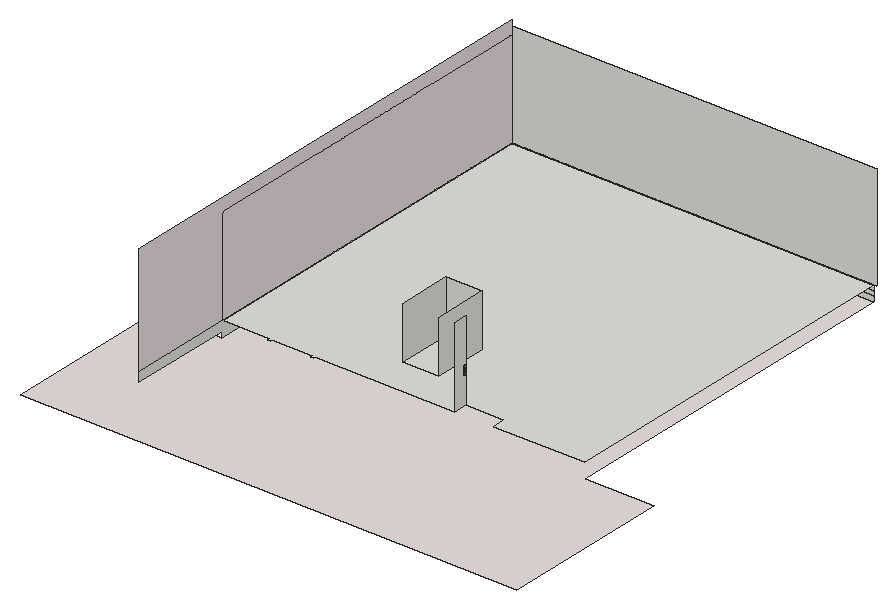
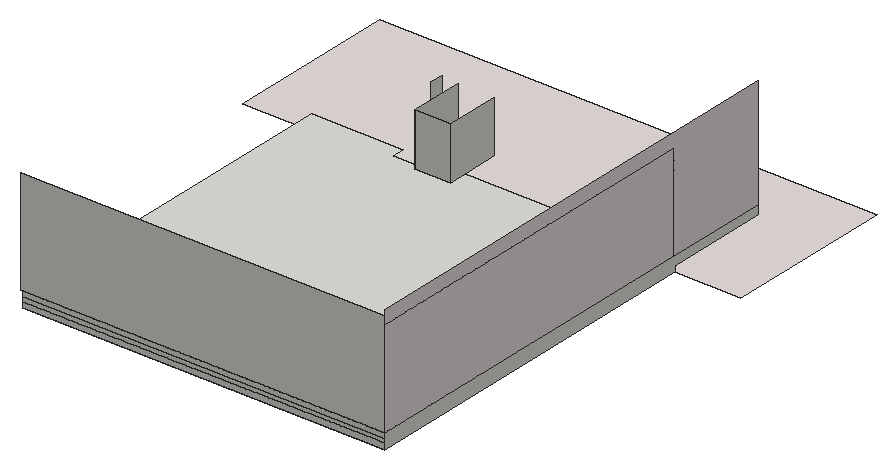
# SketchUp Ruby script. Lengths in inches.
U = 1.inch
M = Sketchup.active_model
def pt(a) = Geom::Point3d.new(a.map { |v| v * U })
def face(e, loops, mat)
  f = e.add_face(loops[0].map { |a| pt(a) })
  loops[1..].each { |l| e.add_face(l.map { |a| pt(a) }).erase! }
  f.material = f.back_material = mat if mat
  f
end
# faces: each face lists its corners as indices into pts; further lists are holes
def faces(e, pts, list, mat = nil) = list.each { |f| face(e, (f[0].is_a?(Array) ? f : [f]).map { |l| l.map { |i| pts[i] } }, mat) }
# xy, xz, yz: faces in a plane at the given z, y or x. An outline is a flat list of corners, or four numbers for a rectangle; further outlines are holes
def ring(l) = l.size == 4 ? [[l[0], l[1]], [l[2], l[1]], [l[2], l[3]], [l[0], l[3]]] : l.each_slice(2).to_a
def flat(e, list, mat, &to3) = list.each { |f| face(e, (f[0].is_a?(Array) ? f : [f]).map { |l| ring(l).map { |u, v| to3.(u, v) } }, mat) }
def xy(e, z, list, mat = nil) = flat(e, list, mat) { |x, y| [x, y, z] }
def xz(e, y, list, mat = nil) = flat(e, list, mat) { |x, z| [x, y, z] }
def yz(e, x, list, mat = nil) = flat(e, list, mat) { |y, z| [x, y, z] }
def lines(e, pts, list) = list.each { |a, b| e.add_line(pt(pts[a]), pt(pts[b])) }
# prism: a flat outline (further loops are holes) pulled along v
def prism(e, loops, v, mat = nil)
  f = face(e, loops, mat); d = Geom::Vector3d.new(v.map { |x| x * U })
  f.pushpull(f.normal.samedirection?(d) ? d.length : -d.length)
end
def box(e, o, s, mat = nil) = prism(e, [[o, [o[0] + s[0], o[1], o[2]], [o[0] + s[0], o[1] + s[1], o[2]], [o[0], o[1] + s[1], o[2]]]], [0, 0, s[2]], mat)
def at(x, y, z, deg = 0) = Geom::Transformation.translation(pt([x, y, z])) * Geom::Transformation.rotation(ORIGIN, Z_AXIS, deg.degrees)
def axes(o, x, y, z) = Geom::Transformation.new([*x, 0, *y, 0, *z, 0, *pt(o).to_a, 1])
def part(name) = M.definitions.add(name)
# library, detail: a bought-in or finely detailed component or shape, given as its bounding box
def library(name, o, s) = part(name).tap { |d| box(d.entities, o, s) }
def detail(e, o, s) = box(e.add_group.entities, o, s)
def put(e, d, t, mat = nil) = e.add_instance(d, t).tap { |i| i.material = mat if mat }
def group(e, t, mat = nil) = e.add_group.tap { |g| g.transformation = t; g.material = mat if mat }.entities
root = M.entities
M.materials.add("Generic\#9").color = [233, 223, 223]
M.materials.add("Material \#1").color = [140, 140, 140]
c1 = library("3DGeom~4_Defintion",[-18.02,-499.97,-221.16],[36.04,1000,262.12])
c2 = part("3DGeom~5_Defintion")
xy(c2.entities,-225.24,[[-0.79,-499.98,-2.33,-499.64,7.45,-496.14],[-0.79,-499.98,7.45,-496.14,1.58,-499.88],[1.58,-499.88,7.45,-496.14,3.84,-499.16],[-2.33,-499.64,7.4,-485.75,7.45,-496.14],[3.84,-499.16,7.45,-496.14,5.85,-497.89],
  [7.45,-496.14,7.4,-485.75,8.24,-487.08],[7.45,-496.14,8.24,-487.08,8.96,-489.34],[7.45,-496.14,8.96,-489.34,9.0625,-491.71],[7.45,-496.14,9.0625,-491.71,8.55,-494.03],[-7.4,-496.08,-8.24,-494.76,2.32,-482.2],
  [-8.24,-494.76,-8.96,-492.5,2.32,-482.2],[-8.96,-492.5,-9.0625,-490.125,2.32,-482.2],[-9.0625,-490.125,-8.55,-487.81,2.32,-482.2],[-8.55,-487.81,-7.45,-485.7,2.32,-482.2],[-7.45,-485.7,-5.85,-483.95,2.32,-482.2],
  [-5.85,-483.95,-3.84,-482.68,2.32,-482.2],[-3.84,-482.68,-1.58,-481.96,2.32,-482.2],[2.32,-482.2,-1.58,-481.96,0.79,-481.86],[0,481.82,-2.35,482.13,-6.92,496.71],[0,481.82,-6.92,496.71,1.55,482.04],
  [-2.35,482.13,-4.55,483.04,-6.92,496.71],[-4.55,483.04,-6.43,484.49,-6.92,496.71],[-6.43,484.49,-7.88,486.37,-6.92,496.71],[6.92,485.12,-1.55,499.8125,7.88,495.47],[6.92,485.12,7.88,495.47,7.88,486.37],
  [-7.88,486.37,-8.79,488.57,-6.92,496.71],[7.88,486.37,7.88,495.47,8.79,488.57],[-8.79,488.57,-9.1,490.92,-6.92,496.71],[8.79,488.57,7.88,495.47,9.1,490.92],[-9.1,490.92,-8.79,493.28,-6.92,496.71],
  [9.1,490.92,7.88,495.47,8.79,493.28],[-8.79,493.28,-7.88,495.47,-6.92,496.71],[7.88,495.47,-1.55,499.8125,0,500.02],[7.88,495.47,0,500.02,2.35,499.71],[7.88,495.47,2.35,499.71,4.55,498.8],
  [7.88,495.47,4.55,498.8,6.43,497.35]],"Material \#1")
xy(c2.entities,-221.57,[[-2.33,-499.64,-5.22,-498.37,7.4,-485.75],[-5.22,-498.37,-7.4,-496.08,5.22,-483.47],[-5.22,-498.37,5.22,-483.47,7.4,-485.75],[-7.4,-496.08,2.32,-482.2,5.22,-483.47],[1.55,482.04,-6.92,496.71,-4.55,498.8],
  [1.55,482.04,-4.55,498.8,4.55,483.04],[4.55,483.04,-4.55,498.8,-1.55,499.8125],[4.55,483.04,-1.55,499.8125,6.92,485.12]],"Material \#1")
xy(c2.entities,38.05,[[-2.33,-499.64,7.4,-485.75,-5.22,-498.37],[-5.22,-498.37,5.22,-483.47,-7.4,-496.08],[-5.22,-498.37,7.4,-485.75,5.22,-483.47],[-7.4,-496.08,5.22,-483.47,2.32,-482.2],[1.55,482.04,-4.55,498.8,-6.92,496.71],
  [1.55,482.04,4.55,483.04,-4.55,498.8],[4.55,483.04,-1.55,499.8125,-4.55,498.8],[4.55,483.04,6.92,485.12,-1.55,499.8125]],"Material \#1")
xy(c2.entities,41.72,[[-0.79,-499.98,7.45,-496.14,-2.33,-499.64],[-0.79,-499.98,1.58,-499.88,7.45,-496.14],[1.58,-499.88,3.84,-499.16,7.45,-496.14],[-2.33,-499.64,7.45,-496.14,7.4,-485.75],[3.84,-499.16,5.85,-497.89,7.45,-496.14],
  [7.45,-496.14,8.24,-487.08,7.4,-485.75],[7.45,-496.14,8.55,-494.03,9.0625,-491.71],[7.45,-496.14,8.96,-489.34,8.24,-487.08],[7.45,-496.14,9.0625,-491.71,8.96,-489.34],[-7.4,-496.08,2.32,-482.2,-8.24,-494.76],
  [-8.24,-494.76,2.32,-482.2,-8.96,-492.5],[-8.96,-492.5,2.32,-482.2,-9.0625,-490.125],[-9.0625,-490.125,2.32,-482.2,-8.55,-487.81],[-8.55,-487.81,2.32,-482.2,-7.45,-485.7],[-7.45,-485.7,2.32,-482.2,-5.85,-483.95],
  [-5.85,-483.95,2.32,-482.2,-3.84,-482.68],[-3.84,-482.68,2.32,-482.2,-1.58,-481.96],[2.32,-482.2,0.79,-481.86,-1.58,-481.96],[0,481.82,-6.92,496.71,-2.35,482.13],[0,481.82,1.55,482.04,-6.92,496.71],
  [-2.35,482.13,-6.92,496.71,-4.55,483.04],[-4.55,483.04,-6.92,496.71,-6.43,484.49],[-6.43,484.49,-6.92,496.71,-7.88,486.37],[6.92,485.12,7.88,495.47,-1.55,499.8125],[6.92,485.12,7.88,486.37,7.88,495.47],
  [-7.88,486.37,-6.92,496.71,-8.79,488.57],[7.88,486.37,8.79,488.57,7.88,495.47],[-8.79,488.57,-6.92,496.71,-9.1,490.92],[8.79,488.57,9.1,490.92,7.88,495.47],[-9.1,490.92,-6.92,496.71,-8.79,493.28],
  [9.1,490.92,8.79,493.28,7.88,495.47],[-8.79,493.28,-6.92,496.71,-7.88,495.47],[7.88,495.47,0,500.02,-1.55,499.8125],[7.88,495.47,2.35,499.71,0,500.02],[7.88,495.47,4.55,498.8,2.35,499.71],
  [7.88,495.47,6.43,497.35,4.55,498.8]],"Material \#1")
c3 = library("3DGeom~12_Defintion",[-95.68,-755.75,-830.03],[191.36,191.37,1000])
c4 = part("3DGeom~10_Defintion")
yz(c4.entities,-68.96,[[-797.08,-844.83,-797.08,-827.59,-922.41,-827.59],[-922.41,-844.83,-797.08,-844.83,-922.41,-827.59]],"Material \#1")
yz(c4.entities,68.97,[[-922.41,-844.83,-797.08,-827.59,-797.08,-844.83],[-922.41,-844.83,-922.41,-827.59,-797.08,-827.59],[-797.08,137.93,-922.41,155.17,-797.08,155.17],[-922.41,137.93,-922.41,155.17,-797.08,137.93]],"Material \#1")
p = [[-15.8,-989.55,-844.83],[-15.8,-989.55,-827.59],[0,-991.38,-827.59],[0,-991.38,-844.83],[15.8,-989.55,-827.59],[15.8,-989.55,-844.83],
  [-30.32,-984.36,-844.83],[-30.32,-984.36,-827.59],[30.31,-984.36,-827.59],[30.31,-984.36,-844.83],[-43.12,-976.21,-844.83],[-43.12,-976.21,-827.59],
  [43.12,-976.21,-827.59],[43.12,-976.21,-844.83],[-53.81,-965.53,-844.83],[-53.81,-965.53,-827.59],[53.8,-965.53,-827.59],[53.8,-965.53,-844.83],
  [-61.95,-952.73,-844.83],[-61.95,-952.73,-827.59],[53.8,-965.53,-827.59],[61.95,-952.73,-827.59],[61.95,-952.73,-844.83],[-67.15,-938.21,-844.83],
  [-67.15,-938.21,-827.59],[67.14,-938.21,-827.59],[67.14,-938.21,-844.83],[-68.96,-922.41,-844.83],[-68.96,-922.41,-827.59],[67.14,-938.21,-827.59],
  [68.97,-922.41,-827.59],[68.97,-922.41,-844.83],[-69.1,-794.86,-844.83],[-69.1,-794.86,-827.59],[-68.96,-797.08,-827.59],[-68.96,-797.08,-844.83],
  [68.97,-797.08,-844.83],[68.97,-797.08,-827.59],[69.11,-794.71,-827.59],[69.11,-794.71,-844.83],[-69.48,-792.73,-844.83],[-69.48,-792.73,-827.59],
  [69.53,-792.51,-827.59],[69.53,-792.51,-844.83],[-70.14,-790.6875,-844.83],[-70.14,-790.6875,-827.59],[70.24,-790.48,-827.59],[70.24,-790.48,-844.83],
  [-71.08,-788.73,-844.83],[-71.08,-788.73,-827.59],[71.22,-788.57,-827.59],[71.22,-788.57,-844.83],[-72.32,-786.86,-844.83],[-72.32,-786.86,-827.59],
  [72.47,-786.78,-827.59],[72.47,-786.78,-844.83],[-73.8,-785.17,-844.83],[-73.8,-785.17,-827.59],[74,-785.04,-827.59],[74,-785.04,-844.83],
  [-75.96,-783.21,-844.83],[-75.96,-783.21,-827.59],[74,-785.04,-827.59],[75.76,-783.39,-827.59],[75.76,-783.39,-844.83],[86.625,-772.95,-827.59],
  [86.61,-772.96,-844.83],[-86.89,-773.25,-844.83],[-86.89,-773.25,-827.59],[-75.96,-783.21,-844.83],[-96.66,-761.8,-844.83],[-96.66,-761.8,-827.59],
  [86.625,-772.95,-827.59],[86.63,-772.94,-844.83],[86.61,-772.96,-844.83],[86.625,-772.95,-827.59],[86.62,-772.95,-827.59],[86.62,-772.95,-827.59],
  [96.31,-761.375,-827.59],[96.31,-761.375,-844.83],[86.63,-772.94,-844.83],[86.625,-772.95,-827.59],[86.62,-772.95,-827.59],[-104.96,-749.18,-844.83],
  [-104.96,-749.18,-827.59],[-96.66,-761.8,-827.59],[-96.66,-761.8,-844.83],[96.31,-761.375,-827.59],[104.62,-748.77,-827.59],[104.62,-748.77,-844.83],
  [-111.64,-735.52,-844.83],[-111.64,-735.52,-827.59],[111.39,-735.21,-827.59],[111.39,-735.21,-844.83],[-116.49,-721.23,-844.83],[-116.49,-721.23,-827.59],
  [116.4375,-720.78,-827.59],[116.4375,-720.78,-844.83],[-119.64,-705.62,-844.83],[-119.64,-705.62,-827.59],[119.6,-705.57,-827.59],[119.6,-705.57,-844.83],
  [-120.6875,-689.65,-844.83],[-120.6875,-689.65,-827.59],[120.69,-689.65,-827.59],[120.69,-689.65,-844.83],[-117.5,-662,-844.83],[-117.5,-662,-827.59],
  [117.5,-662,-827.59],[117.5,-662,-844.83],[-108.41,-636.61,-844.83],[-108.41,-636.61,-827.59],[117.5,-662,-844.83],[108.41,-636.61,-827.59],
  [108.41,-636.61,-844.83],[-93.91,-613.95,-844.83],[-93.91,-613.95,-827.59],[-108.41,-636.61,-827.59],[108.41,-636.61,-844.83],[94.16,-614.19,-827.59],
  [94.16,-614.19,-844.83],[94.16,-614.19,-827.59],[75.46,-595.5,-827.59],[75.46,-595.5,-844.83],[-75.46,-595.5,-844.83],[-75.46,-595.5,-827.59],
  [-93.91,-613.95,-827.59],[-93.91,-613.95,-827.59],[-93.91,-613.95,-844.83],[-53.05,-581.24,-844.83],[-53.05,-581.24,-827.59],[-75.46,-595.5,-827.59],
  [-75.46,-595.5,-844.83],[53.05,-581.24,-827.59],[53.05,-581.24,-844.83],[-27.65,-572.16,-844.83],[-27.65,-572.16,-827.59],[-53.05,-581.24,-827.59],
  [-53.05,-581.24,-844.83],[27.66,-572.16,-827.59],[27.66,-572.16,-844.83],[0,-568.97,-844.83],[0,-568.97,-827.59],[-27.65,-572.16,-827.59],
  [-27.65,-572.16,-844.83],[0,-568.97,-844.83],[-15.8,-989.55,155.17],[0,-991.38,155.17],[0,-991.38,137.93],[-15.8,-989.55,137.93],
  [15.8,-989.55,155.17],[15.8,-989.55,137.93],[-30.32,-984.36,155.17],[-30.32,-984.36,137.93],[30.31,-984.36,155.17],[30.31,-984.36,137.93],
  [-43.125,-976.22,155.17],[-43.125,-976.22,137.93],[43.12,-976.22,155.17],[43.12,-976.22,137.93],[-53.81,-965.53,155.17],[-53.81,-965.53,137.93],
  [53.8,-965.53,155.17],[53.8,-965.53,137.93],[-61.96,-952.73,155.17],[-61.95,-952.73,137.93],[61.95,-952.73,155.17],[61.95,-952.73,137.93],
  [53.8,-965.53,137.93],[-67.15,-938.21,155.17],[-67.15,-938.21,137.93],[67.14,-938.21,155.17],[67.14,-938.21,137.93],[-68.96,-922.41,155.17],
  [-68.96,-922.41,137.93],[68.97,-922.41,155.17],[68.97,-922.41,137.93],[67.14,-938.21,137.93],[-68.97,-797.08,155.17],[-68.97,-797.08,137.93],
  [-69.1,-794.86,155.17],[-69.1,-794.86,137.93],[68.97,-797.08,155.17],[69.11,-794.71,155.17],[69.11,-794.71,137.93],[68.97,-797.08,137.93],
  [-69.48,-792.73,155.17],[-69.48,-792.73,137.93],[69.53,-792.51,155.17],[69.53,-792.51,137.93],[-70.14,-790.6875,155.17],[-70.14,-790.6875,137.93],
  [70.24,-790.48,155.17],[70.24,-790.48,137.93],[-71.08,-788.73,155.17],[-71.08,-788.73,137.93],[71.22,-788.57,155.17],[71.22,-788.57,137.93],
  [-72.32,-786.86,155.17],[-72.32,-786.86,137.93],[72.47,-786.78,155.17],[72.47,-786.78,137.93],[-73.8,-785.17,155.17],[-73.8,-785.17,137.93],
  [74,-785.04,155.17],[74,-785.04,137.93],[-75.96,-783.21,155.17],[-75.96,-783.21,137.93],[75.76,-783.39,155.17],[75.76,-783.39,137.93],
  [74,-785.04,137.93],[86.61,-772.96,155.17],[86.625,-772.95,137.93],[-86.88,-773.25,155.17],[-75.96,-783.21,155.17],[-86.88,-773.25,137.93],
  [-96.66,-761.8,155.17],[-96.66,-761.8,137.93],[86.63,-772.94,155.17],[86.625,-772.95,137.93],[86.61,-772.96,155.17],[86.62,-772.95,137.93],
  [86.625,-772.95,137.93],[96.31,-761.375,155.17],[96.31,-761.375,137.93],[86.62,-772.95,137.93],[86.63,-772.94,155.17],[86.62,-772.95,137.93],
  [86.625,-772.95,137.93],[-104.96,-749.18,155.17],[-96.66,-761.8,155.17],[-96.66,-761.8,137.93],[-104.96,-749.18,137.93],[104.62,-748.77,155.17],
  [104.62,-748.77,137.93],[96.31,-761.375,137.93],[-111.64,-735.52,155.17],[-111.64,-735.52,137.93],[111.39,-735.21,155.17],[111.39,-735.21,137.93],
  [-116.49,-721.23,155.17],[-116.49,-721.23,137.93],[116.4375,-720.78,155.17],[116.4375,-720.78,137.93],[-119.64,-705.62,155.17],[-119.64,-705.62,137.93],
  [119.6,-705.57,155.17],[119.6,-705.57,137.93],[-120.6875,-689.65,155.17],[-120.6875,-689.65,137.93],[120.69,-689.65,155.17],[120.69,-689.65,137.93],
  [-117.5,-662,155.17],[-117.5,-662,137.93],[117.5,-662,155.17],[117.5,-662,137.93],[-108.41,-636.61,155.17],[-108.41,-636.61,137.93],
  [117.5,-662,155.17],[108.41,-636.61,155.17],[108.41,-636.61,137.93],[-93.91,-613.95,155.17],[-108.41,-636.61,137.93],[-93.91,-613.95,137.93],
  [108.41,-636.61,155.17],[94.16,-614.19,155.17],[94.16,-614.19,137.93],[75.46,-595.5,155.17],[75.46,-595.5,137.93],[94.16,-614.19,137.93],
  [-75.46,-595.5,155.17],[-93.91,-613.95,155.17],[-93.91,-613.95,137.93],[-75.46,-595.5,137.93],[-53.05,-581.24,155.17],[-75.46,-595.5,155.17],
  [-75.46,-595.5,137.93],[-53.05,-581.24,137.93],[53.05,-581.24,155.17],[53.05,-581.24,137.93],[-27.65,-572.16,155.17],[-53.05,-581.24,155.17],
  [-53.05,-581.24,137.93],[-27.65,-572.16,137.93],[27.65,-572.16,155.17],[27.65,-572.16,137.93],[0,-568.97,155.17],[-27.65,-572.16,155.17],
  [-27.65,-572.16,137.93],[0,-568.97,137.93],[0,-568.97,155.17]]
faces(c4.entities,p,[[0,1,2],[2,3,0],[3,2,4],[4,5,3],[6,7,1],[1,0,6],[5,4,8],[8,9,5],
  [10,11,7],[7,6,10],[9,8,12],[12,13,9],[14,15,11],[11,10,14],[13,12,16],[16,17,13],
  [18,19,15],[15,14,18],[17,20,21],[21,22,17],[23,24,19],[19,18,23],[22,21,25],[25,26,22],
  [27,28,24],[24,23,27],[26,29,30],[30,31,26],[32,33,34],[34,35,32],[36,37,38],[38,39,36],
  [40,41,33],[33,32,40],[39,38,42],[42,43,39],[44,45,41],[41,40,44],[43,42,46],[46,47,43],
  [48,49,45],[45,44,48],[47,46,50],[50,51,47],[52,53,49],[49,48,52],[51,50,54],[54,55,51],
  [56,57,53],[53,52,56],[55,54,58],[58,59,55],[60,61,57],[57,56,60],[59,62,63],[63,64,59],
  [64,63,65],[65,66,64],[67,68,61],[61,69,67],[70,71,68],[68,67,70],[72,73,66],[74,75,76],
  [73,77,78],[78,79,73],[80,81,82],[83,84,85],[85,86,83],[79,87,88],[88,89,79],[90,91,84],
  [84,83,90],[89,88,92],[92,93,89],[94,95,91],[91,90,94],[93,92,96],[96,97,93],[98,99,95],
  [95,94,98],[97,96,100],[100,101,97],[102,103,99],[99,98,102],[101,100,104],[104,105,101],[106,107,103],
  [103,102,106],[105,104,108],[108,109,105],[110,111,107],[107,106,110],[112,108,113],[113,114,112],[115,116,117],
  [117,110,115],[118,113,119],[119,120,118],[120,121,122],[122,123,120],[124,125,126],[127,128,124],[129,130,131],
  [131,132,129],[123,122,133],[133,134,123],[135,136,137],[137,138,135],[134,133,139],[139,140,134],[141,142,143],
  [143,144,141],[140,139,142],[142,145,140],[146,147,148],[148,149,146],[147,150,151],[151,148,147],[152,146,149],
  [149,153,152],[150,154,155],[155,151,150],[156,152,153],[153,157,156],[154,158,159],[159,155,154],[160,156,157],
  [157,161,160],[158,162,163],[163,159,158],[164,160,161],[161,165,164],[162,166,167],[167,168,162],[169,164,165],
  [165,170,169],[166,171,172],[172,167,166],[173,169,170],[170,174,173],[171,175,176],[176,177,171],[178,173,174],
  [174,179,178],[180,178,179],[179,181,180],[182,183,184],[184,185,182],[186,180,181],[181,187,186],[183,188,189],
  [189,184,183],[190,186,187],[187,191,190],[188,192,193],[193,189,188],[194,190,191],[191,195,194],[192,196,197],
  [197,193,192],[198,194,195],[195,199,198],[196,200,201],[201,197,196],[202,198,199],[199,203,202],[200,204,205],
  [205,201,200],[206,202,203],[203,207,206],[204,208,209],[209,210,204],[208,211,212],[212,209,208],[213,214,207],
  [207,215,213],[216,213,215],[215,217,216],[211,218,219],[220,221,222],[218,223,224],[224,225,218],[226,227,228],
  [229,230,231],[231,232,229],[223,233,234],[234,235,223],[236,229,232],[232,237,236],[233,238,239],[239,234,233],
  [240,236,237],[237,241,240],[238,242,243],[243,239,238],[244,240,241],[241,245,244],[242,246,247],[247,243,242],
  [248,244,245],[245,249,248],[246,250,251],[251,247,246],[252,248,249],[249,253,252],[250,254,255],[255,251,250],
  [256,252,253],[253,257,256],[258,259,260],[260,255,258],[261,256,262],[262,263,261],[264,265,266],[266,260,264],
  [265,267,268],[268,269,265],[270,271,272],[272,273,270],[274,275,276],[276,277,274],[267,278,279],[279,268,267],
  [280,281,282],[282,283,280],[278,284,285],[285,279,278],[286,287,288],[288,289,286],[284,290,289],[289,285,284]],"Material \#1")
c5 = library("3DGeom~14_Defintion",[-102.17,352.37,-727.27],[204.35,204.35,1000])
xy(root,-17.3125,[[0,0,0,192.8125,75.375,192.8125,75.375,607.4375,488.6875,607.4375,488.6875,194.8125,567.25,194.8125,567.25,0]],"Generic\#9")
xy(root,0,[[128.625,192.5,131.625,192.5,131.625,194.8125,177.9375,194.8125,177.9375,192.5,180.9375,192.5,180.9375,194.8125,340.778,194.8125,340.778,210.0625,384.716,210.0625,384.716,194.8125,488.6875,194.8125,488.6875,607.4375,75.375,607.4375,75.375,194.8125,128.625,194.8125]])
xy(root,29.465,[[280.759,194.8125,322.259,256.5625]])
xy(root,40.964,[[347.794,200.864,347.854,201.153,347.794,201.153]],"Material \#1")
xz(root,200.833,[[347.824,40.059,347.754,40.076,347.893,40.076],[347.824,40.059,347.788,40.064,347.754,40.076],[347.754,40.076,347.666,40.53,347.977,40.184],[347.754,40.076,347.67,40.184,347.666,40.53],[347.754,40.076,347.701,40.12,347.67,40.184],
  [347.754,40.076,347.725,40.095,347.701,40.12],[347.701,40.12,347.682,40.15,347.67,40.184],[347.977,40.184,347.663,40.549,347.66,40.554],[347.977,40.184,347.665,40.543,347.663,40.549],[347.977,40.184,347.666,40.536,347.665,40.543],
  [347.67,40.184,347.666,40.221,347.666,40.53],[347.977,40.184,347.666,40.53,347.666,40.536],[347.981,40.221,347.63,40.635,347.668,40.595],[347.981,40.221,347.66,40.554,347.63,40.635],[347.981,40.221,347.668,40.595,347.714,40.565],
  [347.981,40.221,347.714,40.565,347.767,40.546],[347.66,40.554,347.544,40.756,347.6,40.682],[347.66,40.554,347.657,40.56,347.544,40.756],[347.66,40.554,347.6,40.682,347.63,40.635],[347.657,40.56,347.652,40.565,347.544,40.756],
  [347.652,40.565,347.598,40.622,347.544,40.756],[347.652,40.565,347.647,40.57,347.598,40.622],[347.647,40.57,347.621,40.594,347.598,40.622],[347.598,40.622,347.563,40.685,347.544,40.756],[347.598,40.622,347.579,40.652,347.563,40.685],
  [347.6,40.682,347.544,40.756,347.582,40.736],[347.563,40.685,347.551,40.719,347.544,40.756],[347.582,40.736,347.544,40.756,347.575,40.794],[347.544,40.756,347.542,40.794,347.549,40.861],[347.544,40.756,347.549,40.861,347.604,40.975],
  [347.544,40.756,347.582,40.853,347.575,40.794],[347.544,40.756,347.6,40.906,347.582,40.853],[347.544,40.756,347.604,40.975,347.6,40.906],[347.549,40.861,347.571,40.921,347.604,40.975],[347.6,40.906,347.604,40.975,347.63,40.954],
  [347.63,40.954,347.604,40.975,347.668,40.993],[347.604,40.975,347.647,41.02,347.7,41.054],[347.604,40.975,347.7,41.054,347.824,41.083],[347.604,40.975,347.714,41.023,347.668,40.993],[347.604,40.975,347.824,41.083,347.714,41.023],
  [347.714,41.023,347.824,41.083,347.767,41.043],[347.767,41.043,347.824,41.083,347.824,41.049],[347.7,41.054,347.759,41.076,347.824,41.083]],"Material \#1")
xz(root,200.864,[[347.812,40.624,347.836,40.65,347.8,40.65],[347.812,40.624,347.848,40.624,347.836,40.65],[347.8,40.65,347.842,40.658,347.794,40.658],[347.8,40.65,347.836,40.65,347.842,40.658],[347.794,40.658,347.842,40.658,347.842,40.678],
  [347.794,40.658,347.842,40.678,347.794,40.678],[347.794,40.678,347.836,40.686,347.8,40.686],[347.794,40.678,347.842,40.678,347.836,40.686],[347.8,40.686,347.836,40.686,347.848,40.718],[347.8,40.686,347.848,40.718,347.8,40.718],
  [347.8,40.718,347.848,40.718,347.848,40.748],[347.8,40.718,347.848,40.748,347.8,40.748],[347.8,40.748,347.857,40.772,347.791,40.772],[347.8,40.748,347.848,40.748,347.857,40.772],[347.791,40.772,347.857,40.772,347.857,40.796],
  [347.791,40.772,347.857,40.796,347.791,40.796],[347.791,40.796,347.848,40.82,347.8,40.82],[347.791,40.796,347.857,40.796,347.848,40.82],[347.8,40.82,347.854,40.837,347.794,40.837],[347.8,40.82,347.848,40.82,347.854,40.837],
  [347.794,40.837,347.854,40.837,347.854,40.892],[347.794,40.837,347.854,40.892,347.794,40.892],[347.794,40.892,347.847,40.896,347.801,40.896],[347.794,40.892,347.854,40.892,347.847,40.896],[347.801,40.896,347.847,40.896,347.847,40.905],
  [347.801,40.896,347.847,40.905,347.801,40.905],[347.801,40.905,347.854,40.909,347.794,40.909],[347.801,40.905,347.847,40.905,347.854,40.909],[347.794,40.909,347.854,40.909,347.854,40.964],[347.794,40.909,347.854,40.964,347.794,40.964]],"Material \#1")
xz(root,201.082,[[347.824,40.539,347.824,40.548,347.759,40.548],[347.824,40.539,347.886,40.556,347.824,40.548],[347.824,40.539,347.888,40.548,347.886,40.556],[347.759,40.548,347.761,40.556,347.699,40.574],[347.759,40.548,347.824,40.548,347.761,40.556],
  [347.888,40.548,347.944,40.581,347.886,40.556],[347.888,40.548,347.948,40.574,347.944,40.581],[347.761,40.556,347.704,40.581,347.699,40.574],[347.699,40.574,347.704,40.581,347.648,40.614],[347.948,40.574,347.994,40.62,347.944,40.581],
  [347.948,40.574,348,40.614,347.994,40.62],[347.704,40.581,347.654,40.62,347.648,40.614],[347.648,40.614,347.654,40.62,347.608,40.667],[348,40.614,348.032,40.671,347.994,40.62],[348,40.614,348.039,40.667,348.032,40.671],
  [347.654,40.62,347.616,40.671,347.608,40.667],[347.608,40.667,347.616,40.671,347.583,40.728],[348.039,40.667,348.056,40.731,348.032,40.671],[348.039,40.667,348.064,40.728,348.056,40.731],[347.616,40.671,347.592,40.731,347.583,40.728],
  [347.583,40.728,347.592,40.731,347.575,40.794],[348.064,40.728,348.064,40.794,348.056,40.731],[348.064,40.728,348.072,40.794,348.064,40.794],[347.592,40.731,347.583,40.794,347.575,40.794],[347.575,40.794,347.583,40.794,347.583,40.86],
  [347.583,40.794,347.592,40.858,347.583,40.86],[348.064,40.794,348.072,40.794,348.056,40.858],[348.072,40.794,348.064,40.86,348.056,40.858],[347.592,40.858,347.608,40.922,347.583,40.86],[347.592,40.858,347.616,40.918,347.608,40.922],
  [348.056,40.858,348.064,40.86,348.032,40.918],[348.064,40.86,348.039,40.922,348.032,40.918],[347.616,40.918,347.648,40.975,347.608,40.922],[347.616,40.918,347.654,40.969,347.648,40.975],[348.032,40.918,348.039,40.922,347.994,40.969],
  [348.039,40.922,348,40.975,347.994,40.969],[347.654,40.969,347.699,41.015,347.648,40.975],[347.654,40.969,347.704,41.008,347.699,41.015],[347.994,40.969,348,40.975,347.944,41.008],[348,40.975,347.948,41.015,347.944,41.008],
  [347.704,41.008,347.759,41.041,347.699,41.015],[347.704,41.008,347.761,41.032,347.759,41.041],[347.944,41.008,347.948,41.015,347.886,41.032],[347.948,41.015,347.888,41.041,347.886,41.032],[347.761,41.032,347.824,41.049,347.759,41.041],
  [347.761,41.032,347.824,41.041,347.824,41.049],[347.886,41.032,347.888,41.041,347.824,41.041],[347.824,41.041,347.888,41.041,347.824,41.049]],"Material \#1")
xz(root,201.113,[[347.824,37.502,347.824,37.514,347.693,37.514],[347.693,37.514,347.696,37.526,347.571,37.548],[347.693,37.514,347.824,37.514,347.696,37.526],[347.696,37.526,347.575,37.56,347.571,37.548],[347.571,37.548,347.575,37.56,347.458,37.603],
  [347.575,37.56,347.464,37.614,347.458,37.603],[347.458,37.603,347.464,37.614,347.357,37.676],[347.464,37.614,347.365,37.686,347.357,37.676],[347.357,37.676,347.365,37.686,347.269,37.766],[347.365,37.686,347.279,37.774,347.269,37.766],
  [347.824,37.7,347.824,37.713,347.781,37.704],[347.781,37.704,347.783,37.717,347.74,37.716],[347.781,37.704,347.824,37.713,347.783,37.717],[347.74,37.716,347.744,37.728,347.702,37.734],[347.74,37.716,347.783,37.717,347.744,37.728],
  [347.744,37.728,347.708,37.745,347.702,37.734],[347.702,37.734,347.708,37.745,347.669,37.759],[347.708,37.745,347.677,37.768,347.669,37.759],[347.669,37.759,347.677,37.768,347.64,37.788],[347.269,37.766,347.279,37.774,347.201,37.863],
  [347.677,37.768,347.649,37.796,347.64,37.788],[347.279,37.774,347.212,37.87,347.201,37.863],[347.64,37.788,347.649,37.796,347.616,37.823],[347.649,37.796,347.627,37.829,347.616,37.823],[347.616,37.823,347.627,37.829,347.598,37.861],
  [347.627,37.829,347.61,37.866,347.598,37.861],[347.598,37.861,347.61,37.866,347.587,37.903],[347.201,37.863,347.212,37.87,347.144,37.986],[347.61,37.866,347.599,37.905,347.587,37.903],[347.212,37.87,347.156,37.99,347.144,37.986],
  [347.587,37.903,347.599,37.905,347.583,37.943],[347.599,37.905,347.595,37.943,347.583,37.943],[347.583,37.943,347.595,37.943,347.587,37.991],[347.595,37.943,347.599,37.989,347.587,37.991],[347.144,37.986,347.156,37.99,347.111,38.111],
  [347.599,37.989,347.598,38.033,347.587,37.991],[347.599,37.989,347.61,38.029,347.598,38.033],[347.156,37.99,347.123,38.113,347.111,38.111],[347.61,38.029,347.616,38.072,347.598,38.033],[347.61,38.029,347.627,38.065,347.616,38.072],
  [347.627,38.065,347.64,38.106,347.616,38.072],[347.627,38.065,347.649,38.098,347.64,38.106],[347.649,38.098,347.669,38.136,347.64,38.106],[347.649,38.098,347.677,38.126,347.669,38.136],[347.111,38.111,347.123,38.113,347.098,38.249],
  [347.123,38.113,347.111,38.25,347.098,38.249],[347.677,38.126,347.702,38.16,347.669,38.136],[347.677,38.126,347.708,38.149,347.702,38.16],[347.708,38.149,347.74,38.179,347.702,38.16],[347.708,38.149,347.744,38.167,347.74,38.179],
  [347.744,38.167,347.781,38.19,347.74,38.179],[347.744,38.167,347.783,38.178,347.781,38.19],[347.783,38.178,347.824,38.194,347.781,38.19],[347.783,38.178,347.824,38.181,347.824,38.194],[347.098,38.249,347.111,38.25,347.098,46.739],
  [347.111,38.25,347.111,46.738,347.098,46.739]],"Material \#1")
xz(root,201.144,[[347.824,40.059,347.701,40.12,347.754,40.076],[347.824,40.059,347.947,40.12,347.701,40.12],[347.824,40.059,347.754,40.076,347.788,40.064],[347.754,40.076,347.701,40.12,347.725,40.095],[347.947,40.12,347.544,40.756,347.66,40.554],
  [347.947,40.12,347.63,40.635,347.544,40.756],[347.947,40.12,347.668,40.595,347.63,40.635],[347.947,40.12,347.66,40.554,347.663,40.549],[347.947,40.12,347.663,40.549,347.665,40.543],[347.947,40.12,347.665,40.543,347.666,40.536],
  [347.701,40.12,347.666,40.53,347.67,40.184],[347.701,40.12,347.666,40.536,347.666,40.53],[347.701,40.12,347.947,40.12,347.666,40.536],[347.947,40.12,347.714,40.565,347.668,40.595],[347.701,40.12,347.67,40.184,347.682,40.15],
  [347.947,40.12,347.767,40.546,347.714,40.565],[347.67,40.184,347.666,40.53,347.666,40.221],[347.66,40.554,347.544,40.756,347.657,40.56],[347.657,40.56,347.544,40.756,347.652,40.565],[347.652,40.565,347.544,40.756,347.598,40.622],
  [347.652,40.565,347.598,40.622,347.647,40.57],[347.647,40.57,347.598,40.622,347.621,40.594],[347.598,40.622,347.544,40.756,347.563,40.685],[347.598,40.622,347.563,40.685,347.579,40.652],[347.63,40.635,347.6,40.682,347.544,40.756],
  [347.6,40.682,347.582,40.736,347.544,40.756],[347.563,40.685,347.544,40.756,347.551,40.719],[347.582,40.736,347.575,40.794,347.544,40.756],[347.544,40.756,347.549,40.861,347.542,40.794],[347.544,40.756,347.575,40.794,347.582,40.853],
  [347.544,40.756,347.582,40.853,347.604,40.975],[347.544,40.756,347.604,40.975,347.549,40.861],[347.582,40.853,347.6,40.906,347.604,40.975],[347.549,40.861,347.604,40.975,347.571,40.921],[347.6,40.906,347.63,40.954,347.604,40.975],
  [347.63,40.954,347.668,40.993,347.604,40.975],[347.604,40.975,347.668,40.993,347.714,41.023],[347.604,40.975,347.7,41.054,347.647,41.02],[347.604,40.975,347.714,41.023,347.824,41.083],[347.604,40.975,347.824,41.083,347.7,41.054],
  [347.714,41.023,347.767,41.043,347.824,41.083],[347.767,41.043,347.824,41.049,347.824,41.083],[347.7,41.054,347.824,41.083,347.759,41.076]],"Material \#1")
xz(root,201.153,[[347.824,40.567,347.824,40.576,347.766,40.575],[347.824,40.567,347.879,40.583,347.824,40.576],[347.824,40.567,347.881,40.575,347.879,40.583],[347.766,40.575,347.768,40.583,347.713,40.598],[347.766,40.575,347.824,40.576,347.768,40.583],
  [347.881,40.575,347.93,40.605,347.879,40.583],[347.881,40.575,347.934,40.598,347.93,40.605],[347.768,40.583,347.717,40.605,347.713,40.598],[347.713,40.598,347.717,40.605,347.667,40.634],[347.934,40.598,347.974,40.64,347.93,40.605],
  [347.934,40.598,347.98,40.634,347.974,40.64],[347.717,40.605,347.673,40.64,347.667,40.634],[347.667,40.634,347.673,40.64,347.632,40.681],[347.98,40.634,348.008,40.685,347.974,40.64],[347.98,40.634,348.016,40.681,348.008,40.685],
  [347.673,40.64,347.639,40.685,347.632,40.681],[347.632,40.681,347.639,40.685,347.61,40.736],[348.016,40.681,348.03,40.738,348.008,40.685],[348.016,40.681,348.038,40.736,348.03,40.738],[347.639,40.685,347.618,40.738,347.61,40.736],
  [347.61,40.736,347.618,40.738,347.602,40.794],[348.038,40.736,348.037,40.794,348.03,40.738],[348.038,40.736,348.045,40.794,348.037,40.794],[347.618,40.738,347.61,40.794,347.602,40.794],[347.602,40.794,347.61,40.794,347.61,40.853],
  [347.61,40.794,347.618,40.851,347.61,40.853],[348.037,40.794,348.045,40.794,348.03,40.851],[348.045,40.794,348.038,40.853,348.03,40.851],[347.618,40.851,347.632,40.908,347.61,40.853],[347.618,40.851,347.639,40.904,347.632,40.908],
  [348.03,40.851,348.038,40.853,348.008,40.904],[348.038,40.853,348.016,40.908,348.008,40.904],[347.639,40.904,347.667,40.955,347.632,40.908],[347.639,40.904,347.673,40.949,347.667,40.955],[348.008,40.904,348.016,40.908,347.974,40.949],
  [348.016,40.908,347.98,40.955,347.974,40.949],[347.673,40.949,347.713,40.991,347.667,40.955],[347.673,40.949,347.717,40.984,347.713,40.991],[347.974,40.949,347.98,40.955,347.93,40.984],[347.98,40.955,347.934,40.991,347.93,40.984],
  [347.717,40.984,347.766,41.014,347.713,40.991],[347.717,40.984,347.768,41.006,347.766,41.014],[347.93,40.984,347.934,40.991,347.879,41.006],[347.934,40.991,347.881,41.014,347.879,41.006],[347.768,41.006,347.824,41.022,347.766,41.014],
  [347.768,41.006,347.824,41.013,347.824,41.022],[347.879,41.006,347.881,41.014,347.824,41.013],[347.824,41.013,347.881,41.014,347.824,41.022]],"Material \#1")
xz(root,256.5625,[[280.759,29.465,322.259,89.402]])
xz(root,607.4375,[[75.375,-17.3125,488.6875,-10.875],[75.375,-10.875,488.6875,-6],[75.375,-6,488.6875,0],[75.375,0,491.875,120]])
yz(root,75.375,[[192.8125,-17.3125,192.8125,-10.875,75.375,-10.875,75.375,0,607.4375,0,607.4375,-17.3125]])
yz(root,75.375,[[75.375,0,75.375,126,607.4375,126,607.4375,110.75,194.8125,110.75,194.8125,0],[194.8125,0,607.4375,110.75]],"Generic\#9")
yz(root,280.759,[[194.8125,29.465,256.5625,89.402]])
yz(root,322.259,[[194.8125,29.465,256.5625,89.402]])
yz(root,340.778,[[194.8125,0,210.0625,90.9375]])
yz(root,347.794,[[200.864,40.909,200.864,40.964,201.153,40.964]],"Material \#1")
yz(root,347.8,[[200.864,40.686,200.864,40.718,201.153,40.718]],"Material \#1")
p = [[347.797,201.153,40.654],[347.8,200.864,40.65],[347.794,200.864,40.658],[347.797,201.153,40.654],[347.812,201.153,40.624],[347.812,200.864,40.624],
  [347.8,200.864,40.65],[347.797,201.153,40.654],[347.8,200.864,40.748],[347.791,200.864,40.772],[347.791,201.153,40.784],[347.797,201.153,40.682],
  [347.797,201.153,40.654],[347.794,200.864,40.658],[347.794,200.864,40.678],[347.791,201.153,40.784],[347.795,201.153,40.76],[347.8,200.864,40.748],
  [347.797,201.153,40.682],[347.794,200.864,40.678],[347.8,200.864,40.686],[347.795,201.153,40.76],[347.8,201.153,40.718],[347.8,200.864,40.718],
  [347.8,200.864,40.718],[347.8,200.864,40.748],[347.795,201.153,40.76],[347.8,201.153,40.718],[347.797,201.153,40.682],[347.8,200.864,40.686],
  [347.791,200.864,40.772],[347.791,200.864,40.796],[347.795,201.153,40.808],[347.795,201.153,40.808],[347.791,201.153,40.784],[347.791,200.864,40.772],
  [347.797,201.153,40.828],[347.795,201.153,40.808],[347.791,200.864,40.796],[347.794,200.864,40.837],[347.794,200.864,40.892],[347.797,201.153,40.897],
  [347.797,201.153,40.897],[347.794,201.153,40.841],[347.794,200.864,40.837],[347.791,200.864,40.796],[347.8,200.864,40.82],[347.797,201.153,40.828],
  [347.8,200.864,40.82],[347.794,200.864,40.837],[347.794,201.153,40.841],[347.794,201.153,40.841],[347.797,201.153,40.828],[347.8,200.864,40.82],
  [347.794,201.153,40.964],[347.797,201.153,40.897],[347.794,200.864,40.909],[347.851,201.153,40.902],[347.847,200.864,40.896],[347.854,200.864,40.892],
  [347.797,201.153,40.897],[347.801,200.864,40.896],[347.801,200.864,40.905],[347.797,201.153,40.897],[347.794,200.864,40.909],[347.797,201.153,40.897],
  [347.794,200.864,40.892],[347.851,201.153,40.902],[347.854,200.864,40.909],[347.847,200.864,40.905],[347.851,201.153,40.902],[340.778,210.0625,0],
  [340.778,210.0625,-10.875]]
faces(root,p,[[0,1,2],[3,4,5],[5,6,7],[8,9,10],[11,12,13],[13,14,11],[15,16,17],[18,19,20],
  [21,22,23],[24,25,26],[27,28,29],[30,31,32],[33,34,35],[36,37,38],[39,40,41],[42,43,44],
  [45,46,47],[48,49,50],[51,52,53],[54,55,56],[57,58,59],[60,61,62],[63,62,64],[65,66,61],
  [67,68,69],[70,69,58]],"Material \#1")
lines(root,p,[[71,72]])
put(root,c1,axes([347.82,200.83,42.49],[0.0092,0,0],[0,0,0.00943],[0,0.00691,0]),"Material \#1")
put(root,c2,axes([347.82,200.83,42.49],[0.00903,0,0],[0,0,0.00926],[0,0.00678,0]),"Material \#1")
put(root,c3,axes([347.82,200.83,42.49],[0.00251,0,0],[0,0,0.00258],[0,0.00189,0]),"Material \#1")
put(root,c4,axes([347.82,200.83,42.49],[0.0024,0,0],[0,0,0.00246],[0,0.0018,0]),"Material \#1")
put(root,c5,axes([347.82,200.83,42.49],[0.00365,0,0],[0,0,0.00374],[0,0.00274,0]),"Material \#1")
